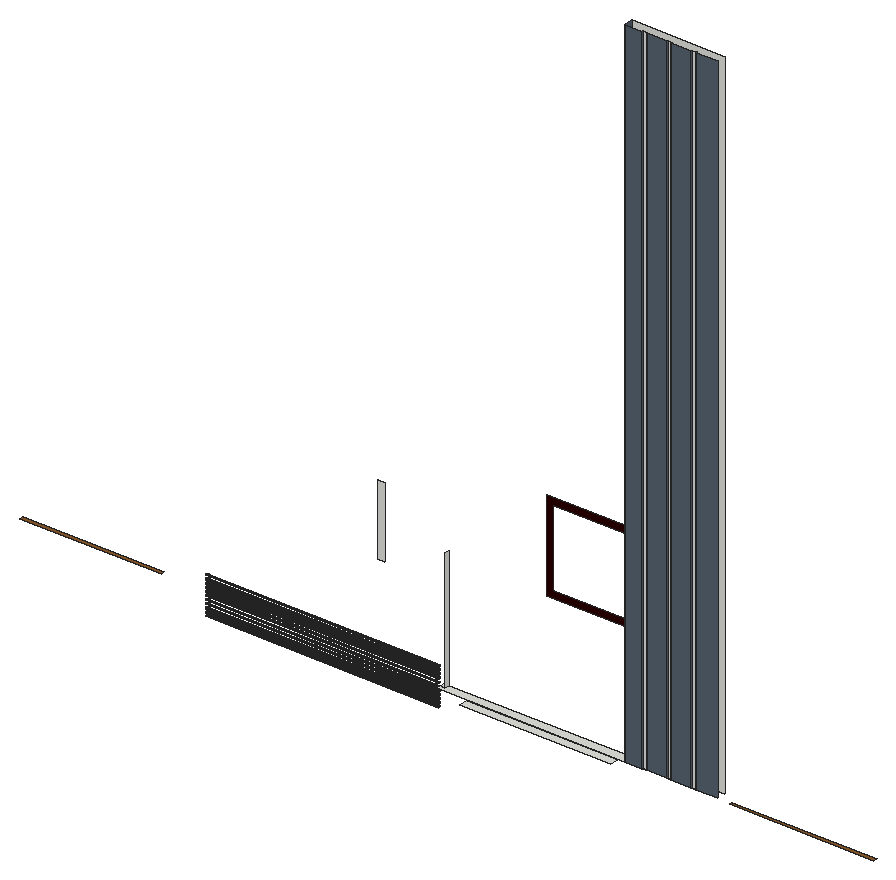
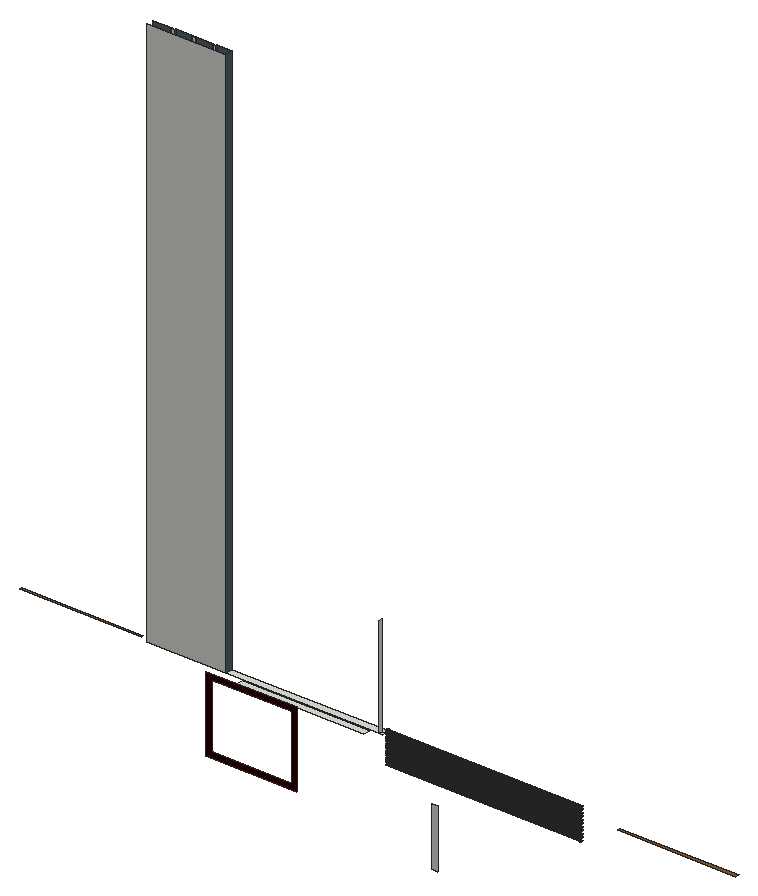
# SketchUp Ruby script. Lengths in inches.
U = 1.inch
M = Sketchup.active_model
def pt(a) = Geom::Point3d.new(a.map { |v| v * U })
def face(e, loops, mat)
  f = e.add_face(loops[0].map { |a| pt(a) })
  loops[1..].each { |l| e.add_face(l.map { |a| pt(a) }).erase! }
  f.material = f.back_material = mat if mat
  f
end
# faces: each face lists its corners as indices into pts; further lists are holes
def faces(e, pts, list, mat = nil) = list.each { |f| face(e, (f[0].is_a?(Array) ? f : [f]).map { |l| l.map { |i| pts[i] } }, mat) }
# xy, xz, yz: faces in a plane at the given z, y or x. An outline is a flat list of corners, or four numbers for a rectangle; further outlines are holes
def ring(l) = l.size == 4 ? [[l[0], l[1]], [l[2], l[1]], [l[2], l[3]], [l[0], l[3]]] : l.each_slice(2).to_a
def flat(e, list, mat, &to3) = list.each { |f| face(e, (f[0].is_a?(Array) ? f : [f]).map { |l| ring(l).map { |u, v| to3.(u, v) } }, mat) }
def xy(e, z, list, mat = nil) = flat(e, list, mat) { |x, y| [x, y, z] }
def xz(e, y, list, mat = nil) = flat(e, list, mat) { |x, z| [x, y, z] }
def yz(e, x, list, mat = nil) = flat(e, list, mat) { |y, z| [x, y, z] }
def lines(e, pts, list) = list.each { |a, b| e.add_line(pt(pts[a]), pt(pts[b])) }
# prism: a flat outline (further loops are holes) pulled along v
def prism(e, loops, v, mat = nil)
  f = face(e, loops, mat); d = Geom::Vector3d.new(v.map { |x| x * U })
  f.pushpull(f.normal.samedirection?(d) ? d.length : -d.length)
end
def box(e, o, s, mat = nil) = prism(e, [[o, [o[0] + s[0], o[1], o[2]], [o[0] + s[0], o[1] + s[1], o[2]], [o[0], o[1] + s[1], o[2]]]], [0, 0, s[2]], mat)
def at(x, y, z, deg = 0) = Geom::Transformation.translation(pt([x, y, z])) * Geom::Transformation.rotation(ORIGIN, Z_AXIS, deg.degrees)
def axes(o, x, y, z) = Geom::Transformation.new([*x, 0, *y, 0, *z, 0, *pt(o).to_a, 1])
def part(name) = M.definitions.add(name)
# library, detail: a bought-in or finely detailed component or shape, given as its bounding box
def library(name, o, s) = part(name).tap { |d| box(d.entities, o, s) }
def detail(e, o, s) = box(e.add_group.entities, o, s)
def put(e, d, t, mat = nil) = e.add_instance(d, t).tap { |i| i.material = mat if mat }
def group(e, t, mat = nil) = e.add_group.tap { |g| g.transformation = t; g.material = mat if mat }.entities
root = M.entities
M.materials.add("[0022_Maroon]").color = [43, 0, 0]
M.materials.add("[0040_Peru]").color = [140, 90, 43]
M.materials.add("[0111_SlateGray]").color = [87, 99, 112]
xy(root,280.8,[[1200,36,1608,60]])
xy(root,297.5,[[1927.54,36,2316,43],[0,60,379.38,69]],"[0040_Peru]")
xy(root,300,[[1140,36,1644,36,1644,60,1152,60,1152,48,1140,48],[1692,36,1704,38],[1758,36,1770,38],[1824,36,1836,38],[1140,48,1152,60]])
xz(root,36,[[1644,300,1692,2076],[1704,300,1758,2076],[1770,300,1824,2076],[1836,300,1896,2076]],"[0111_SlateGray]")
xz(root,38,[[1692,300,1704,2076],[1758,300,1770,2076],[1824,300,1836,2076]])
xz(root,60,[[1644,300,1896,2076]])
xz(root,455.71,[[645.54,254.24,665.16,443.24]])
xz(root,455.71,[[[1098.44,324.3,1390.19,567.56],[1116.44,342.3,1372.19,549.56]]],"[0022_Maroon]")
yz(root,1152,[[48,300,60,624]])
yz(root,1644,[[36,300,60,2076]],"[0111_SlateGray]")
yz(root,1692,[[36,300,38,2076]],"[0111_SlateGray]")
yz(root,1704,[[36,300,38,2076]],"[0111_SlateGray]")
yz(root,1758,[[36,300,38,2076]],"[0111_SlateGray]")
yz(root,1770,[[36,300,38,2076]],"[0111_SlateGray]")
yz(root,1824,[[36,300,38,2076]],"[0111_SlateGray]")
yz(root,1836,[[36,300,38,2076]],"[0111_SlateGray]")
p = [[489.6,72.58,229.2],[489.6,72.52,228.6875],[1116.05,72.52,228.6875],[1116.05,72.58,229.2],[489.6,76.52,228.6875],[489.6,76.45,229.2],
  [1116.05,76.45,229.2],[1116.05,76.52,228.6875],[489.6,72.78,229.6875],[1116.05,72.78,229.6875],[489.6,76.25,229.6875],[1116.05,76.25,229.6875],
  [489.6,73.1,230.1],[1116.05,73.1,230.1],[489.6,75.93,230.1],[1116.05,75.93,230.1],[489.6,73.52,230.42],[1116.05,73.52,230.42],
  [489.6,75.52,230.42],[1116.05,75.52,230.42],[489.6,74,230.62],[1116.05,74,230.62],[489.6,75.03,230.62],[1116.05,75.03,230.62],
  [489.6,74.52,230.6875],[1116.05,74.52,230.6875],[489.6,74,236.75],[489.6,74.52,236.6875],[1116.05,74.52,236.6875],[1116.05,74,236.75],
  [489.6,75.03,236.75],[1116.05,75.03,236.75],[489.6,73.52,236.95],[1116.05,73.52,236.95],[489.6,75.52,236.95],[1116.05,75.52,236.95],
  [489.6,73.1,237.27],[1116.05,73.1,237.27],[489.6,75.93,237.27],[1116.05,75.93,237.27],[489.6,72.78,237.6875],[1116.05,72.78,237.6875],
  [489.6,76.25,237.6875],[1116.05,76.25,237.6875],[489.6,72.58,238.17],[1116.05,72.58,238.17],[489.6,76.45,238.17],[1116.05,76.45,238.17],
  [489.6,72.52,238.6875],[1116.05,72.52,238.6875],[489.6,76.52,238.6875],[1116.05,76.52,238.6875],[489.6,72.58,239.2],[1116.05,72.58,239.2],
  [489.6,76.45,239.2],[1116.05,76.45,239.2],[489.6,72.78,239.6875],[1116.05,72.78,239.6875],[489.6,76.25,239.6875],[1116.05,76.25,239.6875],
  [489.6,73.1,240.1],[1116.05,73.1,240.1],[489.6,75.93,240.1],[1116.05,75.93,240.1],[489.6,73.52,240.42],[1116.05,73.52,240.42],
  [489.6,75.52,240.42],[1116.05,75.52,240.42],[489.6,74,240.62],[1116.05,74,240.62],[489.6,75.03,240.62],[1116.05,75.03,240.62],
  [489.6,74.52,240.6875],[1116.05,74.52,240.6875],[489.6,74,246.75],[489.6,74.52,246.6875],[1116.05,74.52,246.6875],[1116.05,74,246.75],
  [489.6,75.03,246.75],[1116.05,75.03,246.75],[489.6,73.52,246.95],[1116.05,73.52,246.95],[489.6,75.52,246.95],[1116.05,75.52,246.95],
  [489.6,73.1,247.27],[1116.05,73.1,247.27],[489.6,75.93,247.27],[1116.05,75.93,247.27],[489.6,72.78,247.6875],[1116.05,72.78,247.6875],
  [489.6,76.25,247.6875],[1116.05,76.25,247.6875],[489.6,72.58,248.17],[1116.05,72.58,248.17],[489.6,76.45,248.17],[1116.05,76.45,248.17],
  [489.6,72.52,248.6875],[1116.05,72.52,248.6875],[489.6,76.52,248.6875],[1116.05,76.52,248.6875],[489.6,72.58,249.2],[1116.05,72.58,249.2],
  [489.6,76.45,249.2],[1116.05,76.45,249.2],[489.6,72.78,249.6875],[1116.05,72.78,249.6875],[489.6,76.25,249.6875],[1116.05,76.25,249.6875],
  [489.6,73.1,250.1],[1116.05,73.1,250.1],[489.6,75.93,250.1],[1116.05,75.93,250.1],[489.6,73.52,250.42],[1116.05,73.52,250.42],
  [489.6,75.52,250.42],[1116.05,75.52,250.42],[489.6,74,250.62],[1116.05,74,250.62],[489.6,75.03,250.62],[1116.05,75.03,250.62],
  [489.6,74.52,250.6875],[1116.05,74.52,250.6875],[489.6,74,256.75],[489.6,74.52,256.6875],[1116.05,74.52,256.6875],[1116.05,74,256.75],
  [489.6,75.03,256.75],[1116.05,75.03,256.75],[489.6,73.52,256.95],[1116.05,73.52,256.95],[489.6,75.52,256.95],[1116.05,75.52,256.95],
  [489.6,73.1,257.27],[1116.05,73.1,257.27],[489.6,75.93,257.27],[1116.05,75.93,257.27],[489.6,72.78,257.6875],[1116.05,72.78,257.6875],
  [489.6,76.25,257.6875],[1116.05,76.25,257.6875],[489.6,72.58,258.17],[1116.05,72.58,258.17],[489.6,76.45,258.17],[1116.05,76.45,258.17],
  [489.6,72.52,258.6875],[1116.05,72.52,258.6875],[489.6,76.52,258.6875],[1116.05,76.52,258.6875],[489.6,72.58,259.2],[1116.05,72.58,259.2],
  [489.6,76.45,259.2],[1116.05,76.45,259.2],[489.6,72.78,259.6875],[1116.05,72.78,259.6875],[489.6,76.25,259.6875],[1116.05,76.25,259.6875],
  [489.6,73.1,260.1],[1116.05,73.1,260.1],[489.6,75.93,260.1],[1116.05,75.93,260.1],[489.6,73.52,260.42],[1116.05,73.52,260.42],
  [489.6,75.52,260.42],[1116.05,75.52,260.42],[489.6,74,260.62],[1116.05,74,260.62],[489.6,75.03,260.62],[1116.05,75.03,260.62],
  [489.6,74.52,260.6875],[1116.05,74.52,260.6875],[489.6,74,266.75],[489.6,74.52,266.6875],[1116.05,74.52,266.6875],[1116.05,74,266.75],
  [489.6,75.03,266.75],[1116.05,75.03,266.75],[489.6,73.52,266.95],[1116.05,73.52,266.95],[489.6,75.52,266.95],[1116.05,75.52,266.95],
  [489.6,73.1,267.27],[1116.05,73.1,267.27],[489.6,75.93,267.27],[1116.05,75.93,267.27],[489.6,72.78,267.6875],[1116.05,72.78,267.6875],
  [489.6,76.25,267.6875],[1116.05,76.25,267.6875],[489.6,72.58,268.17],[1116.05,72.58,268.17],[489.6,76.45,268.17],[1116.05,76.45,268.17],
  [489.6,72.52,268.6875],[1116.05,72.52,268.6875],[489.6,76.52,268.6875],[1116.05,76.52,268.6875],[489.6,72.58,269.2],[1116.05,72.58,269.2],
  [489.6,76.45,269.2],[1116.05,76.45,269.2],[489.6,72.78,269.6875],[1116.05,72.78,269.6875],[489.6,76.25,269.6875],[1116.05,76.25,269.6875],
  [489.6,73.1,270.1],[1116.05,73.1,270.1],[489.6,75.93,270.1],[1116.05,75.93,270.1],[489.6,73.52,270.42],[1116.05,73.52,270.42],
  [489.6,75.52,270.42],[1116.05,75.52,270.42],[489.6,74,270.62],[1116.05,74,270.62],[489.6,75.03,270.62],[1116.05,75.03,270.62],
  [489.6,74.52,270.6875],[1116.05,74.52,270.6875],[489.6,74,276.75],[489.6,74.52,276.6875],[1116.05,74.52,276.6875],[1116.05,74,276.75],
  [489.6,75.03,276.75],[1116.05,75.03,276.75],[489.6,73.52,276.95],[1116.05,73.52,276.95],[489.6,75.52,276.95],[1116.05,75.52,276.95],
  [489.6,73.1,277.27],[1116.05,73.1,277.27],[489.6,75.93,277.27],[1116.05,75.93,277.27],[489.6,72.78,277.6875],[1116.05,72.78,277.6875],
  [489.6,76.25,277.6875],[1116.05,76.25,277.6875],[489.6,72.58,278.17],[1116.05,72.58,278.17],[489.6,76.45,278.17],[1116.05,76.45,278.17],
  [489.6,72.52,278.6875],[1116.05,72.52,278.6875],[489.6,76.52,278.6875],[1116.05,76.52,278.6875],[489.6,72.58,279.2],[1116.05,72.58,279.2],
  [489.6,76.45,279.2],[1116.05,76.45,279.2],[489.6,72.78,279.6875],[1116.05,72.78,279.6875],[489.6,76.25,279.6875],[1116.05,76.25,279.6875],
  [489.6,73.1,280.1],[1116.05,73.1,280.1],[489.6,75.93,280.1],[1116.05,75.93,280.1],[489.6,73.52,280.42],[1116.05,73.52,280.42],
  [489.6,75.52,280.42],[1116.05,75.52,280.42],[489.6,74,280.62],[1116.05,74,280.62],[489.6,75.03,280.62],[1116.05,75.03,280.62],
  [489.6,74.52,280.6875],[1116.05,74.52,280.6875],[489.6,74,286.75],[489.6,74.52,286.6875],[1116.05,74.52,286.6875],[1116.05,74,286.75],
  [489.6,75.03,286.75],[1116.05,75.03,286.75],[489.6,73.52,286.95],[1116.05,73.52,286.95],[489.6,75.52,286.95],[1116.05,75.52,286.95],
  [489.6,73.1,287.27],[1116.05,73.1,287.27],[489.6,75.93,287.27],[1116.05,75.93,287.27],[489.6,72.78,287.6875],[1116.05,72.78,287.6875],
  [489.6,76.25,287.6875],[1116.05,76.25,287.6875],[489.6,72.58,288.17],[1116.05,72.58,288.17],[489.6,76.45,288.17],[1116.05,76.45,288.17],
  [489.6,72.52,288.6875],[1116.05,72.52,288.6875],[489.6,76.52,288.6875],[1116.05,76.52,288.6875],[489.6,72.58,289.2],[1116.05,72.58,289.2],
  [489.6,76.45,289.2],[1116.05,76.45,289.2],[489.6,72.78,289.6875],[1116.05,72.78,289.6875],[489.6,76.25,289.6875],[1116.05,76.25,289.6875],
  [489.6,73.1,290.1],[1116.05,73.1,290.1],[489.6,75.93,290.1],[1116.05,75.93,290.1],[489.6,73.52,290.42],[1116.05,73.52,290.42],
  [489.6,75.52,290.42],[1116.05,75.52,290.42],[489.6,74,290.62],[1116.05,74,290.62],[489.6,75.03,290.62],[1116.05,75.03,290.62],
  [489.6,74.52,290.6875],[1116.05,74.52,290.6875],[489.6,74,296.75],[489.6,74.52,296.6875],[1116.05,74.52,296.6875],[1116.05,74,296.75],
  [489.6,75.03,296.75],[1116.05,75.03,296.75],[489.6,73.52,296.95],[1116.05,73.52,296.95],[489.6,75.52,296.95],[1116.05,75.52,296.95],
  [489.6,73.1,297.27],[1116.05,73.1,297.27],[489.6,75.93,297.27],[1116.05,75.93,297.27],[489.6,72.78,297.6875],[1116.05,72.78,297.6875],
  [489.6,76.25,297.6875],[1116.05,76.25,297.6875],[489.6,72.58,298.17],[1116.05,72.58,298.17],[489.6,76.45,298.17],[1116.05,76.45,298.17],
  [489.6,72.52,298.6875],[1116.05,72.52,298.6875],[489.6,76.52,298.6875],[1116.05,76.52,298.6875],[489.6,72.58,299.2],[1116.05,72.58,299.2],
  [489.6,76.45,299.2],[1116.05,76.45,299.2],[489.6,72.78,299.6875],[1116.05,72.78,299.6875],[489.6,76.25,299.6875],[1116.05,76.25,299.6875],
  [489.6,73.1,300.1],[1116.05,73.1,300.1],[489.6,75.93,300.1],[1116.05,75.93,300.1],[489.6,73.52,300.42],[1116.05,73.52,300.42],
  [489.6,75.52,300.42],[1116.05,75.52,300.42],[489.6,74,300.62],[1116.05,74,300.62],[489.6,75.03,300.62],[1116.05,75.03,300.62],
  [489.6,74.52,300.6875],[1116.05,74.52,300.6875],[489.6,74,306.75],[489.6,74.52,306.6875],[1116.05,74.52,306.6875],[1116.05,74,306.75],
  [489.6,75.03,306.75],[1116.05,75.03,306.75],[489.6,73.52,306.95],[1116.05,73.52,306.95],[489.6,75.52,306.95],[1116.05,75.52,306.95],
  [489.6,73.1,307.27],[1116.05,73.1,307.27],[489.6,75.93,307.27],[1116.05,75.93,307.27],[489.6,72.78,307.6875],[1116.05,72.78,307.6875],
  [489.6,76.25,307.6875],[1116.05,76.25,307.6875],[489.6,72.58,308.17],[1116.05,72.58,308.17],[489.6,76.45,308.17],[1116.05,76.45,308.17],
  [489.6,72.52,308.6875],[1116.05,72.52,308.6875],[489.6,76.52,308.6875],[1116.05,76.52,308.6875],[489.6,72.58,309.2],[1116.05,72.58,309.2],
  [489.6,76.45,309.2],[1116.05,76.45,309.2],[489.6,72.78,309.6875],[1116.05,72.78,309.6875],[489.6,76.25,309.6875],[1116.05,76.25,309.6875],
  [489.6,73.1,310.1],[1116.05,73.1,310.1],[489.6,75.93,310.1],[1116.05,75.93,310.1],[489.6,73.52,310.42],[1116.05,73.52,310.42],
  [489.6,75.52,310.42],[1116.05,75.52,310.42],[489.6,74,310.62],[1116.05,74,310.62],[489.6,75.03,310.62],[1116.05,75.03,310.62],
  [489.6,74.52,310.6875],[1116.05,74.52,310.6875],[489.6,74,316.75],[489.6,74.52,316.6875],[1116.05,74.52,316.6875],[1116.05,74,316.75],
  [489.6,75.03,316.75],[1116.05,75.03,316.75],[489.6,73.52,316.95],[1116.05,73.52,316.95],[489.6,75.52,316.95],[1116.05,75.52,316.95],
  [489.6,73.1,317.27],[1116.05,73.1,317.27],[489.6,75.93,317.27],[1116.05,75.93,317.27],[489.6,72.78,317.6875],[1116.05,72.78,317.6875],
  [489.6,76.25,317.6875],[1116.05,76.25,317.6875],[489.6,72.58,318.17],[1116.05,72.58,318.17],[489.6,76.45,318.17],[1116.05,76.45,318.17],
  [489.6,72.52,318.6875],[1116.05,72.52,318.6875],[489.6,76.52,318.6875],[1116.05,76.52,318.6875],[489.6,72.58,319.2],[1116.05,72.58,319.2],
  [489.6,76.45,319.2],[1116.05,76.45,319.2],[489.6,72.78,319.6875],[1116.05,72.78,319.6875],[489.6,76.25,319.6875],[1116.05,76.25,319.6875],
  [489.6,73.1,320.1],[1116.05,73.1,320.1],[489.6,75.93,320.1],[1116.05,75.93,320.1],[489.6,73.52,320.42],[1116.05,73.52,320.42],
  [489.6,75.52,320.42],[1116.05,75.52,320.42],[489.6,74,320.62],[1116.05,74,320.62],[489.6,75.03,320.62],[1116.05,75.03,320.62],
  [489.6,74.52,320.6875],[1116.05,74.52,320.6875],[489.6,74,326.75],[489.6,74.52,326.6875],[1116.05,74.52,326.6875],[1116.05,74,326.75],
  [489.6,75.03,326.75],[1116.05,75.03,326.75],[489.6,73.52,326.95],[1116.05,73.52,326.95],[489.6,75.52,326.95],[1116.05,75.52,326.95],
  [489.6,73.1,327.27],[1116.05,73.1,327.27],[489.6,75.93,327.27],[1116.05,75.93,327.27],[489.6,72.78,327.6875],[1116.05,72.78,327.6875],
  [489.6,76.25,327.6875],[1116.05,76.25,327.6875],[489.6,72.58,328.17],[1116.05,72.58,328.17],[489.6,76.45,328.17],[1116.05,76.45,328.17],
  [489.6,72.52,328.6875],[1116.05,72.52,328.6875],[489.6,76.52,328.6875],[1116.05,76.52,328.6875],[489.6,72.58,329.2],[1116.05,72.58,329.2],
  [489.6,76.45,329.2],[1116.05,76.45,329.2],[489.6,72.78,329.6875],[1116.05,72.78,329.6875],[489.6,76.25,329.6875],[1116.05,76.25,329.6875],
  [489.6,73.1,330.1],[1116.05,73.1,330.1],[489.6,75.93,330.1],[1116.05,75.93,330.1],[489.6,73.52,330.42],[1116.05,73.52,330.42],
  [489.6,75.52,330.42],[1116.05,75.52,330.42],[489.6,74,330.62],[1116.05,74,330.62],[489.6,75.03,330.62],[1116.05,75.03,330.62],
  [489.6,74.52,330.6875],[1116.05,74.52,330.6875]]
faces(root,p,[[0,1,2,3],[4,5,6,7],[8,0,3,9],[5,10,11,6],[12,8,9,13],[10,14,15,11],[16,12,13,17],[14,18,19,15],
  [20,16,17,21],[18,22,23,19],[24,20,21,25],[22,24,25,23],[26,27,28,29],[27,30,31,28],[32,26,29,33],[30,34,35,31],
  [36,32,33,37],[34,38,39,35],[40,36,37,41],[38,42,43,39],[44,40,41,45],[42,46,47,43],[48,44,45,49],[46,50,51,47],
  [52,48,49,53],[50,54,55,51],[56,52,53,57],[54,58,59,55],[60,56,57,61],[58,62,63,59],[64,60,61,65],[62,66,67,63],
  [68,64,65,69],[66,70,71,67],[72,68,69,73],[70,72,73,71],[74,75,76,77],[75,78,79,76],[80,74,77,81],[78,82,83,79],
  [84,80,81,85],[82,86,87,83],[88,84,85,89],[86,90,91,87],[92,88,89,93],[90,94,95,91],[96,92,93,97],[94,98,99,95],
  [100,96,97,101],[98,102,103,99],[104,100,101,105],[102,106,107,103],[108,104,105,109],[106,110,111,107],[112,108,109,113],[110,114,115,111],
  [116,112,113,117],[114,118,119,115],[120,116,117,121],[118,120,121,119],[122,123,124,125],[123,126,127,124],[128,122,125,129],[126,130,131,127],
  [132,128,129,133],[130,134,135,131],[136,132,133,137],[134,138,139,135],[140,136,137,141],[138,142,143,139],[144,140,141,145],[142,146,147,143],
  [148,144,145,149],[146,150,151,147],[152,148,149,153],[150,154,155,151],[156,152,153,157],[154,158,159,155],[160,156,157,161],[158,162,163,159],
  [164,160,161,165],[162,166,167,163],[168,164,165,169],[166,168,169,167],[170,171,172,173],[171,174,175,172],[176,170,173,177],[174,178,179,175],
  [180,176,177,181],[178,182,183,179],[184,180,181,185],[182,186,187,183],[188,184,185,189],[186,190,191,187],[192,188,189,193],[190,194,195,191],
  [196,192,193,197],[194,198,199,195],[200,196,197,201],[198,202,203,199],[204,200,201,205],[202,206,207,203],[208,204,205,209],[206,210,211,207],
  [212,208,209,213],[210,214,215,211],[216,212,213,217],[214,216,217,215],[218,219,220,221],[219,222,223,220],[224,218,221,225],[222,226,227,223],
  [228,224,225,229],[226,230,231,227],[232,228,229,233],[230,234,235,231],[236,232,233,237],[234,238,239,235],[240,236,237,241],[238,242,243,239],
  [244,240,241,245],[242,246,247,243],[248,244,245,249],[246,250,251,247],[252,248,249,253],[250,254,255,251],[256,252,253,257],[254,258,259,255],
  [260,256,257,261],[258,262,263,259],[264,260,261,265],[262,264,265,263],[266,267,268,269],[267,270,271,268],[272,266,269,273],[270,274,275,271],
  [276,272,273,277],[274,278,279,275],[280,276,277,281],[278,282,283,279],[284,280,281,285],[282,286,287,283],[288,284,285,289],[286,290,291,287],
  [292,288,289,293],[290,294,295,291],[296,292,293,297],[294,298,299,295],[300,296,297,301],[298,302,303,299],[304,300,301,305],[302,306,307,303],
  [308,304,305,309],[306,310,311,307],[312,308,309,313],[310,312,313,311],[314,315,316,317],[315,318,319,316],[320,314,317,321],[318,322,323,319],
  [324,320,321,325],[322,326,327,323],[328,324,325,329],[326,330,331,327],[332,328,329,333],[330,334,335,331],[336,332,333,337],[334,338,339,335],
  [340,336,337,341],[338,342,343,339],[344,340,341,345],[342,346,347,343],[348,344,345,349],[346,350,351,347],[352,348,349,353],[350,354,355,351],
  [356,352,353,357],[354,358,359,355],[360,356,357,361],[358,360,361,359],[362,363,364,365],[363,366,367,364],[368,362,365,369],[366,370,371,367],
  [372,368,369,373],[370,374,375,371],[376,372,373,377],[374,378,379,375],[380,376,377,381],[378,382,383,379],[384,380,381,385],[382,386,387,383],
  [388,384,385,389],[386,390,391,387],[392,388,389,393],[390,394,395,391],[396,392,393,397],[394,398,399,395],[400,396,397,401],[398,402,403,399],
  [404,400,401,405],[402,406,407,403],[408,404,405,409],[406,408,409,407],[410,411,412,413],[411,414,415,412],[416,410,413,417],[414,418,419,415],
  [420,416,417,421],[418,422,423,419],[424,420,421,425],[422,426,427,423],[428,424,425,429],[426,430,431,427],[432,428,429,433],[430,434,435,431],
  [436,432,433,437],[434,438,439,435],[440,436,437,441],[438,442,443,439],[444,440,441,445],[442,446,447,443],[448,444,445,449],[446,450,451,447],
  [452,448,449,453],[450,454,455,451],[456,452,453,457],[454,456,457,455],[458,459,460,461],[459,462,463,460],[464,458,461,465],[462,466,467,463],
  [468,464,465,469],[466,470,471,467],[472,468,469,473],[470,474,475,471],[476,472,473,477],[474,478,479,475],[480,476,477,481],[478,482,483,479],
  [484,480,481,485],[482,486,487,483],[488,484,485,489],[486,490,491,487],[492,488,489,493],[490,494,495,491],[496,492,493,497],[494,498,499,495],
  [500,496,497,501],[498,502,503,499],[504,500,501,505],[502,504,505,503]])
